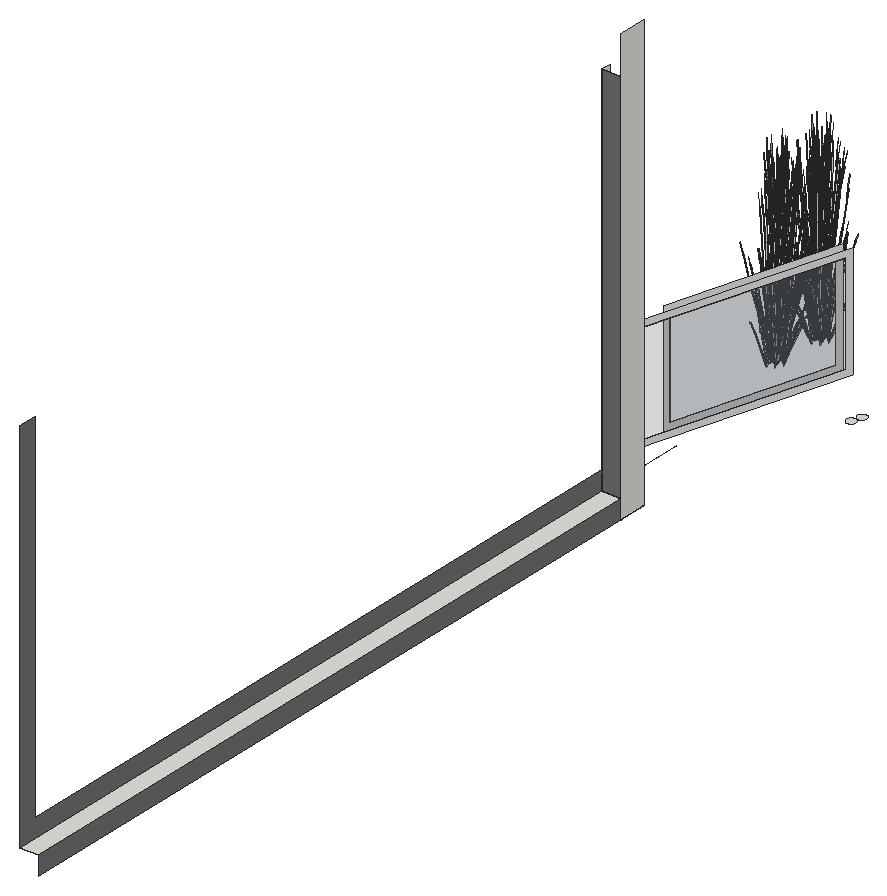
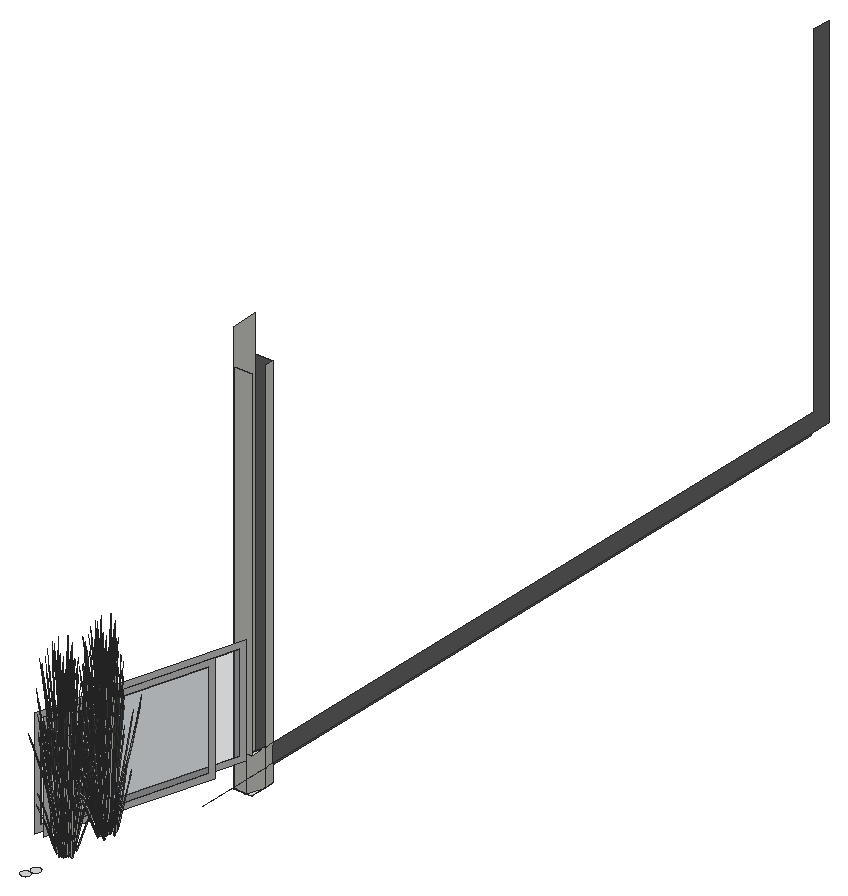
# SketchUp Ruby script. Lengths in inches.
U = 1.inch
M = Sketchup.active_model
def pt(a) = Geom::Point3d.new(a.map { |v| v * U })
def face(e, loops, mat)
  f = e.add_face(loops[0].map { |a| pt(a) })
  loops[1..].each { |l| e.add_face(l.map { |a| pt(a) }).erase! }
  f.material = f.back_material = mat if mat
  f
end
# faces: each face lists its corners as indices into pts; further lists are holes
def faces(e, pts, list, mat = nil) = list.each { |f| face(e, (f[0].is_a?(Array) ? f : [f]).map { |l| l.map { |i| pts[i] } }, mat) }
# xy, xz, yz: faces in a plane at the given z, y or x. An outline is a flat list of corners, or four numbers for a rectangle; further outlines are holes
def ring(l) = l.size == 4 ? [[l[0], l[1]], [l[2], l[1]], [l[2], l[3]], [l[0], l[3]]] : l.each_slice(2).to_a
def flat(e, list, mat, &to3) = list.each { |f| face(e, (f[0].is_a?(Array) ? f : [f]).map { |l| ring(l).map { |u, v| to3.(u, v) } }, mat) }
def xy(e, z, list, mat = nil) = flat(e, list, mat) { |x, y| [x, y, z] }
def xz(e, y, list, mat = nil) = flat(e, list, mat) { |x, z| [x, y, z] }
def yz(e, x, list, mat = nil) = flat(e, list, mat) { |y, z| [x, y, z] }
def lines(e, pts, list) = list.each { |a, b| e.add_line(pt(pts[a]), pt(pts[b])) }
# prism: a flat outline (further loops are holes) pulled along v
def prism(e, loops, v, mat = nil)
  f = face(e, loops, mat); d = Geom::Vector3d.new(v.map { |x| x * U })
  f.pushpull(f.normal.samedirection?(d) ? d.length : -d.length)
end
def box(e, o, s, mat = nil) = prism(e, [[o, [o[0] + s[0], o[1], o[2]], [o[0] + s[0], o[1] + s[1], o[2]], [o[0], o[1] + s[1], o[2]]]], [0, 0, s[2]], mat)
def at(x, y, z, deg = 0) = Geom::Transformation.translation(pt([x, y, z])) * Geom::Transformation.rotation(ORIGIN, Z_AXIS, deg.degrees)
def axes(o, x, y, z) = Geom::Transformation.new([*x, 0, *y, 0, *z, 0, *pt(o).to_a, 1])
def part(name) = M.definitions.add(name)
# library, detail: a bought-in or finely detailed component or shape, given as its bounding box
def library(name, o, s) = part(name).tap { |d| box(d.entities, o, s) }
def detail(e, o, s) = box(e.add_group.entities, o, s)
def put(e, d, t, mat = nil) = e.add_instance(d, t).tap { |i| i.material = mat if mat }
def group(e, t, mat = nil) = e.add_group.tap { |g| g.transformation = t; g.material = mat if mat }.entities
root = M.entities
M.materials.add("Glass_Basic_01").color = [105, 113, 122]
M.materials["Glass_Basic_01"].alpha = 0.25
M.materials.add("LightPink_Translucent").color = [144, 107, 117]
M.materials["LightPink_Translucent"].alpha = 0.75
M.materials.add("M01_Silver_Fog").color = [224, 224, 224]
M.materials.add("M06_Steel_Smoke").color = [114, 114, 114]
c1 = part("blade")
p = [[2.15,0.21,22],[0,0.17,0],[0.09,0.45,0],[2.18,0.31,22],[2.29,0.31,22],[0.38,0.45,0],
  [2.48,0.24,33],[2.49,0.24,33],[2.48,0.22,33]]
faces(c1.entities,p,[[0,1,2,3],[4,5,2,3],[6,3,4,7],[8,0,3,6]])
c2 = part("seeds")
p = [[0.3,-0.1,1.38],[-0.01,-0.03,1.59],[-0.01,-0.03,0.03],[0.14,-0.07,-0.07],[0.29,-0.03,3],[0.15,0.01,3.11]]
faces(c2.entities,p,[[0,1,2,3],[1,0,4,5]],"LightPink_Translucent")
c3 = part("blade with seeds")
put(c3.entities,c1,at(0,0,0))
put(c3.entities,c2,axes([2.4,0.25,30.99],[1.5799,-0.05474,1.17369],[-0.12525,1.92788,0.29478],[-0.07173,-0.02425,1.56792]))
xy(root,510,[[306,231,306,234,307.76,240,312,240,312,231]])
xy(root,510,[[325.27,304.17,325.44,304.17,325.53,304.1875,325.62,304.2,325.7,304.22,325.79,304.25,325.87,304.28,326.03,304.36,326.24,304.51,326.3,304.57,326.42,304.71,326.52,304.85,326.5625,304.93,326.6,305.01,326.66,305.17,326.68,305.26,326.7,305.34,326.72,305.52,326.72,305.61,326.71,305.69,326.7,305.78,326.6875,305.87,326.67,305.95,326.64,306.04,326.61,306.12,326.53,306.28,326.43,306.42,326.375,306.49,326.31,306.55,326.25,306.61,326.18,306.67,326.04,306.77,325.96,306.8125,325.88,306.85,325.72,306.91,325.63,306.93,325.55,306.95,325.37,306.97,325.28,306.97,325.2,306.96,325.11,306.95,325.02,306.9375,324.9375,306.92,324.85,306.89,324.77,306.86,324.61,306.78,324.47,306.68,324.4,306.625,324.33,306.56,324.27,306.5,324.12,306.29,324,306.05,323.98,305.97,323.96,305.88,323.9375,305.8,323.93,305.71,323.92,305.62,323.92,305.53,323.93,305.44,323.9375,305.36,323.95,305.27,323.97,305.1875,324,305.1,324.03,305.02,324.11,304.86,324.26,304.65,324.32,304.58,324.39,304.52,324.6,304.37,324.84,304.25,324.92,304.23,325.01,304.2,325.09,304.1875,325.18,304.18],[326.2,307.35,326.375,307.35,326.46,307.36,326.55,307.38,326.63,307.4,326.72,307.43,326.8,307.46,326.96,307.54,327.17,307.69,327.3,307.82,327.35,307.88,327.4,307.96,327.45,308.03,327.49,308.11,327.53,308.1875,327.56,308.27,327.59,308.35,327.61,308.4375,327.63,308.52,327.65,308.7,327.65,308.79,327.63,308.96,327.62,309.05,327.6,309.13,327.57,309.22,327.54,309.3,327.46,309.46,327.31,309.67,327.25,309.73,327.11,309.85,326.97,309.95,326.89,309.99,326.8125,310.03,326.73,310.0625,326.65,310.09,326.5625,310.11,326.48,310.13,326.3,310.15,326.21,310.15,326.04,310.13,325.95,310.12,325.87,310.1,325.78,310.07,325.7,310.04,325.54,309.96,325.4,309.86,325.33,309.8,325.27,309.74,325.2,309.68,325.05,309.47,325.01,309.39,324.97,309.3125,324.9375,309.23,324.91,309.15,324.89,309.0625,324.87,308.98,324.85,308.8,324.85,308.71,324.87,308.54,324.88,308.45,324.9,308.37,324.93,308.28,324.96,308.2,325.04,308.04,325.14,307.9,325.26,307.76,325.32,307.7,325.53,307.55,325.61,307.5,325.6875,307.47,325.77,307.43,325.85,307.41,325.9375,307.38,326.02,307.37]],"M01_Silver_Fog")
xy(root,510.01,[[306,231,312,240]])
xy(root,516,[[306,0,312,231]])
xy(root,522,[[306,234,307.76,240,306,240]])
xz(root,231,[[306,510.01,312,516]])
xz(root,231,[[306,510,312,510.01],[306,516,312,636]],"M06_Steel_Smoke")
xz(root,240,[[307.76,510,312,510.01],[307.76,510.01,307.76,522,306,522,306,636.01,307.76,636.01,307.76,636,312,636,312,510.01]])
yz(root,306,[[231,510,234,510.01],[234,510,240,510.01],[231,510.01,234,516],[231,516,234,522],[231,522,234,636]])
yz(root,306,[[0,516,231,516,231,522,6,522,6,636,0,636]],"M06_Steel_Smoke")
yz(root,312,[[231,510,240,510.01],[231,510.01,240,648]])
yz(root,312,[[0,510,231,516]],"M06_Steel_Smoke")
p = [[306,234,510],[307.76,240,510],[307.76,240,510.01],[307.76,240,522],[306,234,522],[306,234,516],
  [306,234,510.01],[305.51,243,522],[324.34,307.35,522],[324.34,307.35,558],[305.51,243,558],[323.78,305.43,556],
  [323.78,305.43,524],[306.07,244.92,524],[306.07,244.92,556],[306,255.36,558],[321.22,307.35,558],[321.22,307.35,522],
  [306,255.36,522],[320.65,305.43,556],[306.5625,257.28,556],[306.5625,257.28,524],[320.65,305.43,524],[306,260.5,516]]
faces(root,p,[[0,1,2,3,4,5,6]])
faces(root,p,[[[7,8,9,10],[11,12,13,14]],[[15,16,17,18],[19,20,21,22]]],"M01_Silver_Fog")
faces(root,p,[[12,11,14,13],[20,19,22,21]],"Glass_Basic_01")
lines(root,p,[[23,5]])
put(root,c3,axes([305.04,297.93,524.03],[0.35073,-0.33601,-0.30978],[0.35073,0.33601,0.30978],[0,-0.10823,1.38974]))
put(root,c3,axes([306.62,295.75,524.13],[-0.34721,0.30895,-0.03893],[-0.31814,-0.33837,-0.17649],[-0.0224,-0.09588,0.58215]))
put(root,c3,axes([308.58,315.45,525.33],[0.4342,0.21716,1.51261],[-0.42537,0.46784,0.59816],[-0.19053,-0.27728,1.26806]))
put(root,c3,axes([306.48,298.8,524.36],[0.63506,0.11347,0.45755],[-0.12924,0.64083,0.17955],[-0.09281,-0.06188,1.58856]))
put(root,c3,axes([306.92,311.51,524.77],[0.2621,0.18744,1.1486],[-0.38171,0.11267,0.84392],[-0.08167,-0.14405,0.25299]))
put(root,c3,axes([307.875,314.88,524.21],[-0.30184,-0.45202,-0.44739],[0.45719,-0.31831,0.21531],[-0.09768,-0.05593,1.43643]))
put(root,c3,axes([306.32,298.68,524.72],[-0.24378,0.48527,0.44739],[-0.50654,-0.23354,-0.21531],[0,-0.11186,1.43643]))
put(root,c3,axes([307.12,296.35,526.98],[-0.23981,-0.43789,-0.71045],[0.49365,-0.24404,0.08574],[-0.05608,-0.21158,1.00501]))
put(root,c3,axes([306.14,299.82,524.47],[0.53992,-0.14294,0.17642],[0.13332,0.53195,0.35086],[-0.04815,-0.07751,1.60407]))
put(root,c3,axes([306.83,299.91,524.2],[-0.50654,-0.24178,0],[0.24378,-0.50239,0],[0,0,1.62707]))
put(root,c3,axes([308.01,300.51,524.375],[0.31414,0.53965,0],[-0.52557,0.30095,-0.51607],[-0.1197,0.06854,1.63711]))
put(root,c3,axes([307.92,315.14,524.4375],[0.13317,-0.63814,-0.23429],[0.63143,0.11124,0.51271],[-0.11033,-0.08813,1.5644]))
put(root,c3,axes([308.15,315.29,524.62],[-0.09693,0.48062,0.1448],[-0.47357,-0.08343,-0.41347],[-0.08619,-0.04935,1.26744]))
put(root,c3,axes([307.75,299.85,524.47],[0.14515,-0.53522,0.17642],[0.53115,0.15146,0.35086],[-0.09175,0.00261,1.60407]))
put(root,c3,axes([307.5,299.14,524.62],[0.37121,0.32357,0.1448],[-0.30963,0.36505,-0.41347],[-0.08619,0.04935,1.26744]))
put(root,c3,axes([306.31,313.95,524.02],[0,-0.53854,-0.49651],[0.56215,0,0],[0,-0.12266,1.57504]))
put(root,c3,axes([306.55,314.45,524.48],[0,0.53854,0.49651],[-0.56215,0,0],[0,-0.12266,1.57504]))
put(root,c3,axes([307.37,298.74,524.3],[-0.46736,-0.46353,-0.06131],[0.46764,-0.46381,0],[-0.01632,-0.01619,1.75571]))
put(root,c3,axes([307.49,298.91,524.72],[0.54562,-0.03324,0.44739],[0.04934,0.55185,-0.21531],[-0.09768,0.05593,1.43643]))
put(root,c3,axes([307.625,300.17,524.33],[0.62903,0.17504,0.30756],[-0.15737,0.62568,-0.36492],[-0.10411,0.07831,1.64885]))
put(root,c3,axes([306.71,295.375,523.49],[-0.08428,0.0194,1.76342],[-0.46606,-0.21841,-0.26939],[0.00782,-0.18218,0.30037]))
put(root,c3,axes([307.9,300.14,524.48],[0.47024,-0.26927,0.49651],[0.28107,0.48284,0],[-0.1071,0.06133,1.57504]))
put(root,c3,axes([307.78,314.57,524.67],[-0.56585,-0.25696,-0.29095],[0.27246,-0.54236,-0.50002],[-0.01778,-0.13316,1.59708]))
put(root,c3,axes([307.17,295.97,526.53],[0.15148,-0.41415,-0.35414],[0.44193,0.12079,0.4572],[-0.04052,-0.16674,0.87481]))
put(root,c3,axes([306.43,298.21,524.36],[0.21845,0.6022,0.45755],[-0.62418,0.20941,0.17955],[0.00763,-0.11065,1.58856]))
put(root,c3,axes([306.33,298.13,524.21],[0.24378,-0.48527,-0.44739],[0.50654,0.23354,0.21531],[0,-0.11186,1.43643]))
put(root,c3,axes([306.95,299.7,524.2],[-0.16394,-0.4643,0],[0.46814,-0.1626,0],[0,0,1.54371]))
put(root,c3,axes([306.35,300.68,523.49],[0.08132,-0.0293,1.76342],[0.48914,0.1613,-0.26939],[0.0143,0.18179,0.30037]))
put(root,c3,axes([306.46,300.84,526.53],[-0.15148,0.41415,-0.35414],[-0.44193,-0.12079,0.4572],[0.04052,0.16674,0.87481]))
put(root,c3,axes([307.52,314.03,524.1],[-0.20635,-0.55225,-0.69835],[0.59439,-0.19889,-0.18329],[-0.02281,-0.18701,1.54149]))
put(root,c3,axes([308.45,312.29,526.68],[-0.49392,-0.135,-0.51099],[0.1693,-0.46287,-0.3958],[-0.04529,-0.18636,0.97773]))
put(root,c3,axes([306.55,313.96,524.03],[0.35073,-0.33601,-0.30978],[0.35073,0.33601,0.30978],[0,-0.10823,1.38974]))
put(root,c3,axes([307.61,298.78,524.21],[-0.24378,0.48527,-0.44739],[-0.50654,-0.23354,0.21531],[0,0.11186,1.43643]))
put(root,c3,axes([308.13,311.79,524.13],[-0.34721,0.30895,-0.03893],[-0.31814,-0.33837,-0.17649],[-0.0224,-0.09588,0.58215]))
put(root,c3,axes([307.99,314.83,524.36],[0.63506,0.11347,0.45755],[-0.12924,0.64083,0.17955],[-0.09281,-0.06188,1.58856]))
put(root,c3,axes([308.58,298.49,524.47],[-0.39477,-0.39228,0.17642],[0.39783,-0.38049,0.35086],[-0.0436,0.08011,1.60407]))
put(root,c3,axes([307.21,298.26,524.21],[0,-0.62313,0],[0.62828,0,0],[0,0,1.79456]))
put(root,c3,axes([307.83,314.72,524.72],[-0.24378,0.48527,0.44739],[-0.50654,-0.23354,-0.21531],[0,-0.11186,1.43643]))
put(root,c3,axes([308.63,312.38,526.98],[-0.23981,-0.43789,-0.71045],[0.49365,-0.24404,0.08574],[-0.05608,-0.21158,1.00501]))
put(root,c3,axes([306.63,298.375,524.43],[0.56613,0.26102,0.24065],[-0.27246,0.54236,0.50002],[0,-0.12502,1.60543]))
put(root,c3,axes([307.53,298.51,524.29],[0,0.62282,-0.05637],[-0.62828,0,0],[0,0.01957,1.79368]))
put(root,c3,axes([306.45,298.01,524.72],[-0.54562,0.03324,0.44739],[-0.04934,-0.55185,-0.21531],[0.09768,-0.05593,1.43643]))
put(root,c3,axes([306.19,297.0625,524.47],[-0.14515,0.53522,0.17642],[-0.53115,-0.15146,0.35086],[0.09175,-0.00261,1.60407]))
put(root,c3,axes([307.23,299.72,524.29],[0.21845,0.61869,-0.06012],[-0.62418,0.21679,0],[0.00763,0.02161,1.72173]))
put(root,c3,axes([307.65,315.86,524.47],[0.53992,-0.14294,0.17642],[0.13332,0.53195,0.35086],[-0.04815,-0.07751,1.60407]))
put(root,c3,axes([305.93,296.4,524.375],[-0.31414,-0.53965,0],[0.52557,-0.30095,-0.51607],[0.1197,-0.06854,1.63711]))
put(root,c3,axes([306.51,300.47,526.98],[0.23981,0.43789,-0.71045],[-0.49365,0.24404,0.08574],[0.05608,0.21158,1.00501]))
put(root,c3,axes([309.03,298.9,524.2],[-0.62797,-0.00431,-0.04976],[0,-0.6019,0.49943],[-0.01973,0.13702,1.58352]))
put(root,c3,axes([307.8,297.09,524.47],[-0.53992,0.14294,0.17642],[-0.13332,-0.53195,0.35086],[0.04815,0.07751,1.60407]))
put(root,c3,axes([309.26,315.89,524.47],[0.14515,-0.53522,0.17642],[0.53115,0.15146,0.35086],[-0.09175,0.00261,1.60407]))
put(root,c3,axes([307.25,295.1,524.77],[0.06446,0.31404,1.1486],[-0.35756,-0.17393,0.84392],[0.03848,-0.1608,0.25299]))
put(root,c3,axes([308.88,314.78,524.3],[-0.46736,-0.46353,-0.06131],[0.46764,-0.46381,0],[-0.01632,-0.01619,1.75571]))
put(root,c3,axes([306.91,297.87,524.36],[-0.4166,0.48873,0.45755],[-0.49494,-0.43142,0.17955],[0.10044,-0.04877,1.58856]))
put(root,c3,axes([307.625,298.64,524.21],[0.35073,0.34786,0],[-0.35073,0.34786,0],[0,0,1.69266]))
put(root,c3,axes([307.62,298.23,524.72],[0.24378,-0.48527,0.44739],[0.50654,0.23354,-0.21531],[0,0.11186,1.43643]))
put(root,c3,axes([307.41,299.92,524.2],[0.50654,0.24178,0],[-0.24378,0.50239,0],[0,0,1.74954]))
put(root,c3,axes([308.22,311.41,523.49],[-0.08428,0.0194,1.76342],[-0.46606,-0.21841,-0.26939],[0.00782,-0.18218,0.30037]))
put(root,c3,axes([306.6875,300.56,526.68],[0.49392,0.135,-0.51099],[-0.1693,0.46287,-0.3958],[0.04529,0.18636,0.97773]))
put(root,c3,axes([307.46,298.12,524.38],[-0.63506,-0.11347,0.49198],[0.12924,-0.64083,0.19306],[0.09281,0.06188,1.70813]))
put(root,c3,axes([308.68,312.01,526.53],[0.15148,-0.41415,-0.35414],[0.44193,0.12079,0.4572],[-0.04052,-0.16674,0.87481]))
put(root,c3,axes([307.9375,314.24,524.36],[0.21845,0.6022,0.45755],[-0.62418,0.20941,0.17955],[0.00763,-0.11065,1.58856]))
put(root,c3,axes([307.84,314.17,524.21],[0.24378,-0.48527,-0.44739],[0.50654,0.23354,0.21531],[0,-0.11186,1.43643]))
put(root,c3,axes([308.46,315.73,524.2],[-0.16394,-0.4643,0],[0.46814,-0.1626,0],[0,0,1.54371]))
put(root,c3,axes([308.9,298.99,524.03],[-0.35073,0.33601,-0.30978],[-0.35073,-0.33601,0.30978],[0,0.10823,1.38974]))
put(root,c3,axes([307.9,298.93,524.09],[0.18424,0.49308,-0.69212],[-0.53071,0.17758,-0.18165],[0.02036,0.16697,1.52773]))
put(root,c3,axes([307.64,298.4,524.21],[0.56215,0,0],[0,0.55754,0],[0,0,1.78407]))
put(root,c3,axes([307.1,297.79,524.72],[-0.30184,-0.45202,0.44739],[0.45719,-0.31831,-0.21531],[0.09768,0.05593,1.43643]))
put(root,c3,axes([306.55,297.89,524.67],[-0.05855,-0.61451,-0.29095],[0.60981,-0.03716,-0.50002],[0.10738,-0.08185,1.59708]))
put(root,c3,axes([307.83,298.34,524.62],[0.46814,-0.15705,0.1448],[0.16394,0.44848,-0.41347],[0,0.0987,1.26744]))
put(root,c3,axes([308.01,296.61,526.68],[-0.35968,-0.36185,-0.51099],[0.37996,-0.3169,-0.3958],[0.05473,-0.18385,0.97773]))
put(root,c3,axes([307.67,298.38,524.67],[0.56585,0.25696,-0.29095],[-0.27246,0.54236,-0.50002],[0.01778,0.13316,1.59708]))
put(root,c3,axes([310.09,314.52,524.47],[-0.39477,-0.39228,0.17642],[0.39783,-0.38049,0.35086],[-0.0436,0.08011,1.60407]))
put(root,c3,axes([306.47,296.53,524.03],[0.46876,0.13325,-0.30978],[-0.11803,0.46926,0.30978],[0.0945,-0.05411,1.38974]))
put(root,c3,axes([308.72,314.3,524.21],[0,-0.62313,0],[0.62828,0,0],[0,0,1.79456]))
put(root,c3,axes([308.14,314.41,524.43],[0.56613,0.26102,0.24065],[-0.27246,0.54236,0.50002],[0,-0.12502,1.60543]))
put(root,c3,axes([307.77,295.97,524.59],[-0.14282,0.10901,1.43002],[-0.42773,-0.19079,-0.30754],[0.07929,-0.23728,0.61141]))
put(root,c3,axes([307.96,314.05,524.72],[-0.54562,0.03324,0.44739],[-0.04934,-0.55185,-0.21531],[0.09768,-0.05593,1.43643]))
put(root,c3,axes([308.9,298.5,524.48],[0,-0.53854,0.49651],[0.56215,0,0],[0,0.12266,1.57504]))
put(root,c3,axes([309.14,299,524.02],[0,0.53854,-0.49651],[-0.56215,0,0],[0,0.12266,1.57504]))
put(root,c3,axes([306.36,296.32,524.02],[0.47024,-0.26927,-0.49651],[0.28107,0.48284,0],[0.1071,-0.06133,1.57504]))
put(root,c3,axes([307.7,313.1,524.47],[-0.14515,0.53522,0.17642],[-0.53115,-0.15146,0.35086],[0.09175,-0.00261,1.60407]))
put(root,c3,axes([306.97,299.6,525.875],[-0.11485,-0.17291,1.71376],[0.53072,-0.14557,0.13857],[0.11995,0.27145,0.73262]))
put(root,c3,axes([307.3,297.66,524.62],[0.09693,-0.48062,0.1448],[0.47357,0.08343,-0.41347],[0.08619,0.04935,1.26744]))
put(root,c3,axes([307.44,312.4375,524.375],[-0.31414,-0.53965,0],[0.52557,-0.30095,-0.51607],[0.1197,-0.06854,1.63711]))
put(root,c3,axes([307.97,296.82,524.48],[-0.47024,-0.26927,0.49651],[0.28107,-0.48284,0],[0.1071,0.06133,1.57504]))
put(root,c3,axes([308.12,296.77,526.98],[0.01307,-0.49815,-0.71045],[0.55054,0.03346,0.08574],[0.0581,-0.21104,1.00501]))
put(root,c3,axes([309.31,313.13,524.47],[-0.53992,0.14294,0.17642],[-0.13332,-0.53195,0.35086],[0.04815,0.07751,1.60407]))
put(root,c3,axes([307.5625,299.63,524.18],[0.5275,-0.18273,-0.19198],[0.18536,0.52636,0.00008],[0.05823,-0.0202,1.73897]))
put(root,c3,axes([308.76,311.13,524.77],[0.06446,0.31404,1.1486],[-0.35756,-0.17393,0.84392],[0.03848,-0.1608,0.25299]))
put(root,c3,axes([308.43,313.9,524.36],[-0.4166,0.48873,0.45755],[-0.49494,-0.43142,0.17955],[0.10044,-0.04877,1.58856]))
put(root,c3,axes([309.14,314.67,524.21],[0.35073,0.34786,0],[-0.35073,0.34786,0],[0,0,1.69266]))
put(root,c3,axes([307.57,298.07,524.21],[0.30184,0.45202,-0.44739],[-0.45719,0.31831,0.21531],[0.09768,0.05593,1.43643]))
put(root,c3,axes([308.97,314.15,524.38],[-0.63506,-0.11347,0.49198],[0.12924,-0.64083,0.19306],[0.09281,0.06188,1.70813]))
put(root,c3,axes([308.35,296.47,526.53],[0.33997,-0.28354,-0.35414],[0.32182,0.32376,0.4572],[0.04897,-0.1645,0.87481]))
put(root,c3,axes([308.43,300.12,524.77],[-0.2829,-0.15485,1.1486],[0.36529,-0.15734,0.84392],[0.09853,0.13328,0.25299]))
put(root,c3,axes([307.42,299.95,524.59],[0.00887,-0.17852,1.43002],[0.42372,-0.19941,-0.30754],[0.1308,0.21367,0.61141]))
put(root,c3,axes([306.92,297.42,524.06],[0.33843,-0.40479,-0.62353],[0.42041,0.36705,-0.16365],[0.13561,-0.10098,1.37633]))
put(root,c3,axes([309.15,314.43,524.21],[0.56215,0,0],[0,0.55754,0],[0,0,1.78407]))
put(root,c3,axes([308.61,313.82,524.72],[-0.30184,-0.45202,0.44739],[0.45719,-0.31831,-0.21531],[0.09768,0.05593,1.43643]))
put(root,c3,axes([308.06,313.93,524.67],[-0.05855,-0.61451,-0.29095],[0.60981,-0.03716,-0.50002],[0.10738,-0.08185,1.59708]))
put(root,c3,axes([309.52,312.64,526.68],[-0.35968,-0.36185,-0.51099],[0.37996,-0.3169,-0.3958],[0.05473,-0.18385,0.97773]))
put(root,c3,axes([308.4,297.07,524.03],[0.11803,0.46926,-0.30978],[-0.46876,0.13325,0.30978],[0.0945,0.05411,1.38974]))
put(root,c3,axes([309.28,298.59,524.375],[0.62828,0,0],[0,0.6019,-0.51607],[0,0.13709,1.63711]))
put(root,c3,axes([307.25,297.81,524.67],[0.5073,-0.35754,-0.29095],[0.33735,0.5052,-0.50002],[0.12516,0.05131,1.59708]))
put(root,c3,axes([307.98,312.57,524.03],[0.46876,0.13325,-0.30978],[-0.11803,0.46926,0.30978],[0.0945,-0.05411,1.38974]))
put(root,c3,axes([308.47,300.82,524.67],[-0.3222,-0.01689,1.0506],[0.21278,-0.35872,0.58006],[0.12729,0.12745,0.8241]))
put(root,c3,axes([309.28,312,524.59],[-0.14282,0.10901,1.43002],[-0.42773,-0.19079,-0.30754],[0.07929,-0.23728,0.61141]))
put(root,c3,axes([307.5,296.52,525.875],[-0.09355,0.18511,1.71376],[-0.39247,-0.38307,0.13857],[0.17705,-0.23875,0.73262]))
put(root,c3,axes([307.87,312.35,524.02],[0.47024,-0.26927,-0.49651],[0.28107,0.48284,0],[0.1071,-0.06133,1.57504]))
put(root,c3,axes([308.8125,313.69,524.62],[0.09693,-0.48062,0.1448],[0.47357,0.08343,-0.41347],[0.08619,0.04935,1.26744]))
put(root,c3,axes([305.97,297.5,523.59],[-0.49456,0.21561,1.28929],[-0.15741,-0.61865,0.50096],[0.30369,0.01029,1.46642]))
put(root,c3,axes([309.48,312.86,524.48],[-0.47024,-0.26927,0.49651],[0.28107,-0.48284,0],[0.1071,0.06133,1.57504]))
put(root,c3,axes([309.63,312.81,526.98],[0.01307,-0.49815,-0.71045],[0.55054,0.03346,0.08574],[0.0581,-0.21104,1.00501]))
put(root,c3,axes([309.07,315.67,524.18],[0.5275,-0.18273,-0.19198],[0.18536,0.52636,0.00008],[0.05823,-0.0202,1.73897]))
put(root,c3,axes([307.79,300.33,526.68],[0.4958,-0.12802,-0.51099],[0.08673,0.48481,-0.3958],[0.13317,0.13893,0.97773]))
put(root,c3,axes([308.24,296.54,524.375],[0.31414,-0.53965,0],[0.52557,0.30095,-0.51607],[0.1197,0.06854,1.63711]))
put(root,c3,axes([308.77,296.3,523.49],[-0.0752,-0.04243,1.76342],[-0.19317,-0.47398,-0.26939],[0.13031,-0.12863,0.30037]))
put(root,c3,axes([308.53,296.86,524.02],[0.47024,0.26927,-0.49651],[-0.28107,0.48284,0],[0.1071,0.06133,1.57504]))
put(root,c3,axes([308.51,300.7,523.49],[0.03661,-0.07775,1.76342],[0.46087,-0.22898,-0.26939],[0.13972,0.11851,0.30037]))
put(root,c3,axes([308.76,297.44,526.68],[-0.12908,-0.49174,-0.51099],[0.48882,-0.08602,-0.3958],[0.14008,-0.13208,0.97773]))
put(root,c3,axes([309.61,299.98,525.93],[-0.09617,-0.45271,-0.03492],[0.45453,-0.10408,-0.15832],[0.09492,0.0287,0.52218]))
put(root,c3,axes([309.86,312.51,526.53],[0.33997,-0.28354,-0.35414],[0.32182,0.32376,0.4572],[0.04897,-0.1645,0.87481]))
put(root,c3,axes([307.84,297.9,524.06],[0.52267,0.08829,-0.62353],[-0.11029,0.54463,-0.16365],[0.15598,0.06599,1.37633]))
put(root,c3,axes([310.07,298.22,524.26],[-0.31151,-0.34437,-0.06488],[0.34117,-0.31553,-0.29416],[0.09667,-0.02221,0.97024]))
put(root,c3,axes([308.43,313.46,524.06],[0.33843,-0.40479,-0.62353],[0.42041,0.36705,-0.16365],[0.13561,-0.10098,1.37633]))
put(root,c3,axes([309.36,296.46,524.77],[-0.16736,0.27414,1.1486],[-0.14385,-0.36832,0.84392],[0.13822,-0.09229,0.25299]))
put(root,c3,axes([309.91,313.1,524.03],[0.11803,0.46926,-0.30978],[-0.46876,0.13325,0.30978],[0.0945,0.05411,1.38974]))
put(root,c3,axes([308.76,313.85,524.67],[0.5073,-0.35754,-0.29095],[0.33735,0.5052,-0.50002],[0.12516,0.05131,1.59708]))
put(root,c3,axes([307.74,299.0625,525.875],[-0.18664,-0.09279,1.71376],[0.38624,-0.38925,0.13857],[0.24072,0.1756,0.73262]))
put(root,c3,axes([309.01,312.56,525.875],[-0.09355,0.18511,1.71376],[-0.39247,-0.38307,0.13857],[0.17705,-0.23875,0.73262]))
put(root,c3,axes([309.12,297.49,526.53],[0.43736,-0.07697,-0.35414],[0.11549,0.43998,0.4572],[0.12533,-0.11818,0.87481]))
put(root,c3,axes([308.77,297.64,526.98],[0.26246,-0.42493,-0.71045],[0.45991,0.30199,0.08574],[0.15671,-0.15395,1.00501]))
put(root,c3,axes([308.76,299.93,526.53],[0.28589,0.33718,-0.35414],[-0.32644,0.31919,0.4572],[0.16586,0.04856,0.87481]))
put(root,c3,axes([307.48,313.53,523.59],[-0.49456,0.21561,1.28929],[-0.15741,-0.61865,0.50096],[0.30369,0.01029,1.46642]))
put(root,c3,axes([309.76,312.57,524.375],[0.31414,-0.53965,0],[0.52557,0.30095,-0.51607],[0.1197,0.06854,1.63711]))
put(root,c3,axes([310.28,312.34,523.49],[-0.0752,-0.04243,1.76342],[-0.19317,-0.47398,-0.26939],[0.13031,-0.12863,0.30037]))
put(root,c3,axes([310.04,312.9,524.02],[0.47024,0.26927,-0.49651],[-0.28107,0.48284,0],[0.1071,0.06133,1.57504]))
put(root,c3,axes([308.98,298.53,526.68],[0.13612,-0.48987,-0.51099],[0.46669,0.16791,-0.3958],[0.1879,-0.04492,0.97773]))
put(root,c3,axes([310.27,313.48,526.68],[-0.12908,-0.49174,-0.51099],[0.48882,-0.08602,-0.3958],[0.14008,-0.13208,0.97773]))
put(root,c3,axes([310.15,298.85,524.77],[-0.31044,0.08891,1.1486],[0.14613,-0.36744,0.84392],[0.16469,0.02514,0.25299]))
put(root,c3,axes([309.15,297.25,524.59],[-0.1795,-0.01595,1.43002],[-0.18389,-0.42791,-0.30754],[0.22051,-0.12105,0.61141]))
put(root,c3,axes([309.27,298.76,526.53],[0.41757,0.15024,-0.35414],[-0.12179,0.4383,0.4572],[0.16812,-0.04019,0.87481]))
put(root,c3,axes([309.36,313.93,524.06],[0.52267,0.08829,-0.62353],[-0.11029,0.54463,-0.16365],[0.15598,0.06599,1.37633]))
put(root,c3,axes([311.58,314.25,524.26],[-0.31151,-0.34437,-0.06488],[0.34117,-0.31553,-0.29416],[0.09667,-0.02221,0.97024]))
put(root,c3,axes([308.46,299.7,526.98],[0.50227,0.01297,-0.71045],[-0.03373,0.54602,0.08574],[0.21278,0.05762,1.00501]))
put(root,c3,axes([310.87,312.5,524.77],[-0.16736,0.27414,1.1486],[-0.14385,-0.36832,0.84392],[0.13822,-0.09229,0.25299]))
put(root,c3,axes([309.48,298.67,523.98],[-0.32361,0.06463,1.41583],[-0.05151,-0.51444,0.08104],[0.22666,-0.07786,0.80566]))
put(root,c3,axes([309.83,298.34,523.49],[-0.02626,-0.08176,1.76342],[0.18213,-0.47826,-0.26939],[0.18372,-0.00688,0.30037]))
put(root,c3,axes([308.13,298.21,525.875],[-0.20841,0.0122,1.71376],[0.13825,-0.52864,0.13857],[0.297,0.0327,0.73262]))
put(root,c3,axes([308.89,298.71,526.98],[0.44151,-0.23785,-0.71045],[0.24605,0.4896,0.08574],[0.21333,-0.05562,1.00501]))
put(root,c3,axes([310.625,313.53,526.53],[0.43736,-0.07697,-0.35414],[0.11549,0.43998,0.4572],[0.12533,-0.11818,0.87481]))
put(root,c3,axes([310.28,313.67,526.98],[0.26246,-0.42493,-0.71045],[0.45991,0.30199,0.08574],[0.15671,-0.15395,1.00501]))
put(root,c3,axes([309.57,299.4375,524.59],[-0.12101,-0.13245,1.43002],[0.15744,-0.43816,-0.30754],[0.24483,0.05936,0.61141]))
put(root,c3,axes([310.49,314.57,526.68],[0.13612,-0.48987,-0.51099],[0.46669,0.16791,-0.3958],[0.1879,-0.04492,0.97773]))
put(root,c3,axes([311.67,314.88,524.77],[-0.31044,0.08891,1.1486],[0.14613,-0.36744,0.84392],[0.16469,0.02514,0.25299]))
put(root,c3,axes([310.66,313.28,524.59],[-0.1795,-0.01595,1.43002],[-0.18389,-0.42791,-0.30754],[0.22051,-0.12105,0.61141]))
put(root,c3,axes([310.78,314.79,526.53],[0.41757,0.15024,-0.35414],[-0.12179,0.4383,0.4572],[0.16812,-0.04019,0.87481]))
put(root,c3,axes([310.99,314.71,523.98],[-0.32361,0.06463,1.41583],[-0.05151,-0.51444,0.08104],[0.22666,-0.07786,0.80566]))
put(root,c3,axes([311.35,314.37,523.49],[-0.02626,-0.08176,1.76342],[0.18213,-0.47826,-0.26939],[0.18372,-0.00688,0.30037]))
put(root,c3,axes([309.64,314.25,525.875],[-0.20841,0.0122,1.71376],[0.13825,-0.52864,0.13857],[0.297,0.0327,0.73262]))
put(root,c3,axes([310.4,314.75,526.98],[0.44151,-0.23785,-0.71045],[0.24605,0.4896,0.08574],[0.21333,-0.05562,1.00501]))
